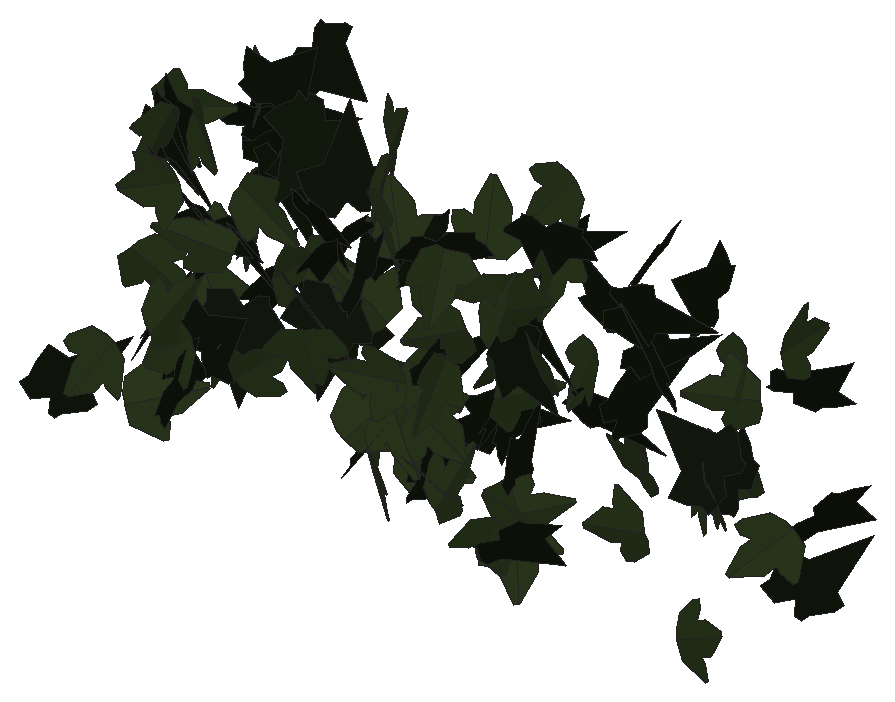
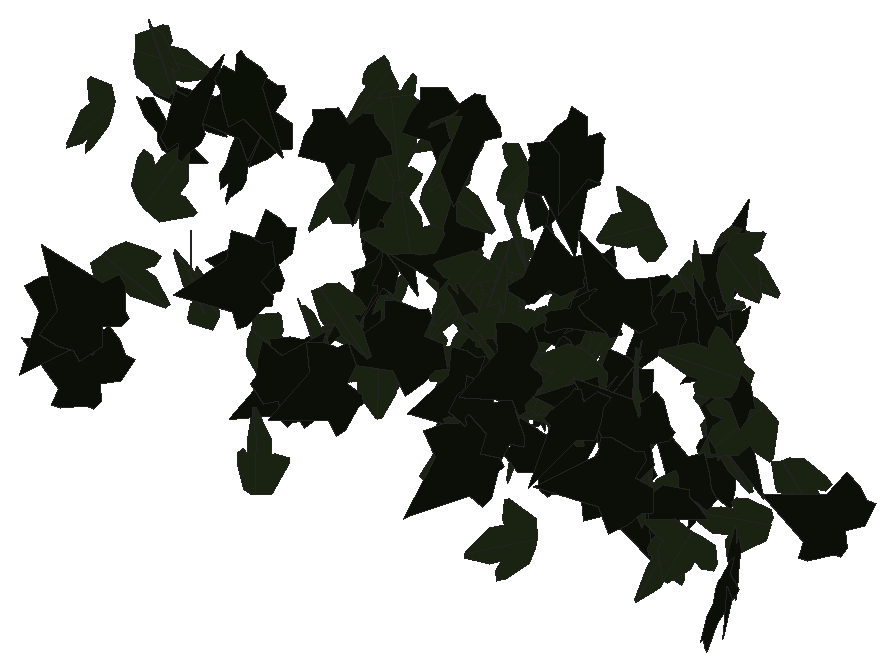
# SketchUp Ruby script. Lengths in inches.
U = 1.inch
M = Sketchup.active_model
def pt(a) = Geom::Point3d.new(a.map { |v| v * U })
def face(e, loops, mat)
  f = e.add_face(loops[0].map { |a| pt(a) })
  loops[1..].each { |l| e.add_face(l.map { |a| pt(a) }).erase! }
  f.material = f.back_material = mat if mat
  f
end
# faces: each face lists its corners as indices into pts; further lists are holes
def faces(e, pts, list, mat = nil) = list.each { |f| face(e, (f[0].is_a?(Array) ? f : [f]).map { |l| l.map { |i| pts[i] } }, mat) }
# xy, xz, yz: faces in a plane at the given z, y or x. An outline is a flat list of corners, or four numbers for a rectangle; further outlines are holes
def ring(l) = l.size == 4 ? [[l[0], l[1]], [l[2], l[1]], [l[2], l[3]], [l[0], l[3]]] : l.each_slice(2).to_a
def flat(e, list, mat, &to3) = list.each { |f| face(e, (f[0].is_a?(Array) ? f : [f]).map { |l| ring(l).map { |u, v| to3.(u, v) } }, mat) }
def xy(e, z, list, mat = nil) = flat(e, list, mat) { |x, y| [x, y, z] }
def xz(e, y, list, mat = nil) = flat(e, list, mat) { |x, z| [x, y, z] }
def yz(e, x, list, mat = nil) = flat(e, list, mat) { |y, z| [x, y, z] }
def lines(e, pts, list) = list.each { |a, b| e.add_line(pt(pts[a]), pt(pts[b])) }
# prism: a flat outline (further loops are holes) pulled along v
def prism(e, loops, v, mat = nil)
  f = face(e, loops, mat); d = Geom::Vector3d.new(v.map { |x| x * U })
  f.pushpull(f.normal.samedirection?(d) ? d.length : -d.length)
end
def box(e, o, s, mat = nil) = prism(e, [[o, [o[0] + s[0], o[1], o[2]], [o[0] + s[0], o[1] + s[1], o[2]], [o[0], o[1] + s[1], o[2]]]], [0, 0, s[2]], mat)
def at(x, y, z, deg = 0) = Geom::Transformation.translation(pt([x, y, z])) * Geom::Transformation.rotation(ORIGIN, Z_AXIS, deg.degrees)
def axes(o, x, y, z) = Geom::Transformation.new([*x, 0, *y, 0, *z, 0, *pt(o).to_a, 1])
def part(name) = M.definitions.add(name)
# library, detail: a bought-in or finely detailed component or shape, given as its bounding box
def library(name, o, s) = part(name).tap { |d| box(d.entities, o, s) }
def detail(e, o, s) = box(e.add_group.entities, o, s)
def put(e, d, t, mat = nil) = e.add_instance(d, t).tap { |i| i.material = mat if mat }
def group(e, t, mat = nil) = e.add_group.tap { |g| g.transformation = t; g.material = mat if mat }.entities
root = M.entities
M.materials.add("efeu1").color = [18, 25, 13]
M.materials.add("efeu2").color = [43, 57, 29]
c1 = part("ivyleaf_9")
p = [[1.54,2.16,1.25],[1.36,2.04,1.19],[-0.21,0.99,0.68],[-0.71,1.11,0.82],[-0.85,0.86,0.67],[-0.8,0.17,0.21],
  [-0.9,-0.01,0.1],[-0.67,-0.16,-0.02],[-0.08,-0.08,-0.05],[-0.03,-0.6,-0.4],[0.65,-0.88,-0.66],[0.83,-0.6,-0.49],
  [1.29,-0.42,-0.43],[1.8125,-0.07,-0.26],[1.21,0.44,0.15]]
faces(c1.entities,p,[[0,1,2,3,4,5,6,7,8,9,10,11,12,13,14]],"efeu1")
c2 = part("ivyleaf_10")
p = [[0,0.5,-0.03],[-0.0625,2.02,-0.43],[-0.19,2.01,-0.46],[-0.54,1.05,-0.29],[-0.52,0.625,-0.18],[-0.83,0.76,-0.28],
  [-1.16,0.64,-0.33],[-1.15,0.33,-0.24],[-0.77,-0.39,0.02],[-0.3,-0.51,0.16],[0.04,-0.48,0.23],[-0.02,2.01,-0.4375],
  [-0.06,2.01,-0.43],[0.04,-0.49,0.23],[0.67,-0.49,0.14],[1.38,0.36,-0.2],[1.375,0.51,-0.24],[0.81,0.65,-0.19],
  [0.62,0.59,-0.15],[0.6,1.09,-0.28],[0.5,1.23,-0.31]]
faces(c2.entities,p,[[0,1,2,3,4,5,6,7,8,9,10],[11,12,0,13,14,15,16,17,18,19,20]],"efeu2")
put(root,c1,axes([43.35,221.53,207.23],[0.45432,0.02484,-0.2073],[-0.20694,-0.0122,-0.455],[-0.02766,0.49923,-0.00081]))
put(root,c2,axes([46.76,221.66,202.9],[-0.31271,-0.38378,-0.07017],[0.04449,0.05425,-0.49505],[0.3876,-0.31586,0.00022]))
put(root,c1,axes([47.18,221.57,206.24],[0.2418,-0.30239,-0.31637],[-0.16835,0.26937,-0.38613],[0.40397,0.29325,0.02846]))
put(root,c2,axes([44.68,221.74,204.64],[0.03954,-0.01046,-0.49832],[-0.49747,0.03022,-0.04011],[0.03095,0.49898,-0.00802]))
put(root,c2,axes([45.54,221.95,204.97],[0.04865,0.35182,-0.35193],[-0.06472,-0.34613,-0.35497],[-0.4934,0.08009,0.01186]))
put(root,c2,axes([47.03,221.4,206.375],[0.00393,0.31947,-0.3846],[0.00224,0.3846,0.31949],[0.49998,-0.00424,0.00159]))
put(root,c2,axes([50.32,221.9,202.12],[0.19082,-0.11068,-0.44871],[0.37864,-0.2409,0.22044],[-0.26499,-0.42393,-0.00812]))
put(root,c2,axes([46.91,221.98,203.04],[-0.10747,0.34806,0.34249],[0.09946,-0.32774,0.36428],[0.47808,0.14643,0.00121]))
put(root,c2,axes([43.1,221.73,204.78],[-0.4383,-0.2361,-0.04633],[0.04211,0.01951,-0.49784],[0.23689,-0.44031,0.00278]))
put(root,c1,axes([43.75,221.61,206.77],[-0.04412,0.49157,-0.08007],[0.00277,-0.08014,-0.49353],[-0.49804,-0.04399,0.00434]))
put(root,c1,axes([51.04,221.76,205.26],[-0.41065,-0.14113,-0.24789],[-0.22963,-0.09422,0.43404],[-0.16923,0.47032,0.01257]))
put(root,c2,axes([39.1,221.83,203.12],[0.43051,-0.06518,-0.24579],[-0.2439,0.03088,-0.43539],[0.07194,0.49477,-0.00521]))
put(root,c1,axes([47.08,221.5,202.84],[0.33902,0.34548,0.12535],[0.08795,0.08933,-0.48403],[-0.35684,0.35024,-0.0002]))
put(root,c2,axes([40.33,221.78,206.49],[0.2199,-0.04325,-0.44696],[-0.42776,0.13124,-0.22315],[0.13662,0.48053,0.02072]))
put(root,c2,axes([46.66,222.07,205.55],[-0.10134,-0.41992,-0.25178],[0.01766,-0.26009,0.42666],[-0.4893,0.07759,0.06754]))
put(root,c1,axes([38.39,221.56,202.29],[-0.00687,-0.00369,0.49994],[0.45435,0.20859,0.00779],[-0.20862,0.4544,0.00049]))
put(root,c2,axes([45.56,221.92,206.91],[0.23152,0.42123,-0.1377],[-0.07114,-0.11802,-0.48064],[-0.43742,0.24215,0.00529]))
put(root,c2,axes([47.23,221.54,206.88],[-0.03633,-0.19491,-0.45901],[0.08664,0.45076,-0.19826],[0.49109,-0.09395,0.00102]))
put(root,c2,axes([47.11,221.5625,205.34],[-0.05853,-0.08283,-0.48961],[0.25997,0.41492,-0.10127],[0.42307,-0.26642,-0.0055]))
put(root,c2,axes([44.1,221.71,203.66],[0.2989,0.1501,-0.37166],[0.33203,0.167,0.33447],[0.22454,-0.44675,0.00016]))
put(root,c2,axes([45.74,222.01,205.75],[-0.18904,-0.08032,0.45587],[-0.4238,-0.16801,-0.20534],[0.18616,-0.46403,-0.00456]))
put(root,c2,axes([44.62,221.91,203.94],[0.41171,0.09001,0.26905],[0.25718,0.08181,-0.42091],[-0.11979,0.48498,0.02107]))
put(root,c2,axes([50.84,221.77,204.9375],[-0.35148,0.26985,0.23161],[-0.18644,0.13748,-0.4431],[-0.30283,-0.39784,0.00398]))
put(root,c1,axes([44.375,221.77,203.52],[-0.18094,0.46067,0.07101],[-0.03614,0.06208,-0.49481],[-0.46471,-0.1842,0.01083]))
put(root,c1,axes([46.89,221.98,205.07],[-0.2203,0.42523,-0.1437],[0.06215,-0.12963,-0.47889],[-0.44453,-0.22886,0.00426]))
put(root,c1,axes([44.19,221.77,206.21],[-0.29069,0.1354,-0.38363],[-0.34489,0.16804,0.32064],[0.21576,0.45103,-0.0043]))
put(root,c2,axes([45.32,221.82,204.18],[0.13161,0.36904,0.31062],[0.08006,0.3008,-0.39129],[-0.47568,0.15273,0.02008]))
put(root,c2,axes([46.59,222.11,206.79],[-0.31601,-0.38523,0.04169],[-0.02644,-0.03223,-0.49826],[0.38657,-0.31711,0]))
put(root,c2,axes([47.34,221.95,205.92],[-0.41901,0.18221,0.20305],[-0.18826,0.07623,-0.45689],[-0.19745,-0.45934,0.00473]))
put(root,c1,axes([45.48,221.93,207.2],[0.23324,0.40175,-0.18493],[-0.10128,-0.15499,-0.46446],[-0.43051,0.25412,0.00907]))
put(root,c1,axes([40.24,222.29,206.05],[0.3681,-0.32071,0.10794],[-0.07679,0.07616,0.48816],[-0.32956,-0.37596,0.00681]))
put(root,c2,axes([40.96,222.26,205.4],[0.12781,0.09886,0.47317],[-0.36591,-0.30004,0.16152],[0.31588,-0.38756,-0.00435]))
put(root,c2,axes([45.38,221.74,206.62],[-0.00296,0.20045,0.45805],[-0.08688,0.45089,-0.19787],[-0.49239,-0.08076,0.03216]))
put(root,c2,axes([41.72,222.11,206.57],[0.23522,0.03018,0.44018],[0.42187,0.13072,-0.23439],[-0.12923,0.48166,0.03603]))
put(root,c2,axes([40.2,221.82,204.07],[0.05586,0.16556,-0.46848],[0.13592,0.44835,0.17465],[0.47792,-0.14687,0.00508]))
put(root,c2,axes([51.05,222.35,206.31],[-0.03612,0.02668,0.49798],[-0.42886,-0.25647,-0.01737],[0.25451,-0.42838,0.04141]))
put(root,c1,axes([42.47,222.17,205.31],[0.45795,-0.19849,-0.02968],[-0.02765,0.01082,-0.49912],[0.19878,0.45879,-0.00106]))
put(root,c2,axes([46.86,221.93,203.03],[-0.00418,-0.00227,-0.49998],[0.36037,0.34657,-0.00458],[0.34658,-0.36039,-0.00126]))
put(root,c2,axes([46.74,222.22,202.44],[0.37811,0.32562,0.03165],[0.02367,0.02102,-0.499],[-0.3263,0.37885,0.00048]))
put(root,c1,axes([44.89,222,203.18],[0.45553,0.07713,-0.19117],[-0.2049,0.11841,-0.44045],[-0.02266,0.47961,0.13949]))
put(root,c2,axes([40.26,222.2,203.57],[0.35093,-0.12137,-0.33484],[-0.30124,0.14962,-0.36995],[0.19,0.46139,0.03189]))
put(root,c1,axes([51.08,222.1,204.9],[-0.1559,0.16793,0.4444],[-0.30212,0.32592,-0.22914],[-0.36664,-0.33997,-0.00015]))
put(root,c1,axes([40.39,221.97,203.05],[-0.05734,0.04993,-0.49419],[-0.34391,0.35494,0.07576],[0.35838,0.3486,-0.00636]))
put(root,c2,axes([45.51,221.96,202.85],[0.0448,0.20704,-0.45291],[0.06869,0.44782,0.21151],[0.49323,-0.08117,0.01168]))
put(root,c1,axes([40.89,222.28,205.79],[0.25536,0.2511,-0.34892],[-0.24352,-0.24994,-0.35809],[-0.35425,0.35282,-0.00535]))
put(root,c1,axes([45.28,221.99,204.74],[0.09046,0.08246,0.48479],[0.33107,0.35426,-0.12203],[-0.3636,0.34308,0.0095]))
put(root,c2,axes([44.73,222.29,204.32],[-0.42024,0.02271,0.26997],[-0.26948,0.01618,-0.42085],[-0.02785,-0.49922,-0.00136]))
put(root,c1,axes([39.98,222.38,204.125],[-0.25861,0.39169,-0.17233],[0.09915,-0.14103,-0.46934],[-0.41628,-0.27692,-0.00473]))
put(root,c2,axes([39.62,222.65,206.95],[0.0227,-0.41266,0.28142],[0.0645,-0.27693,-0.41128],[0.4953,0.05498,0.04066]))
put(root,c1,axes([46.85,222.09,203.54],[-0.001,-0.10231,0.48942],[0.14173,0.46929,0.09839],[-0.47949,0.13893,0.02807]))
put(root,c2,axes([44.93,222.18,204.7],[0.127,0.3496,0.33414],[0.0784,0.32602,-0.3709],[-0.47721,0.1466,0.02799]))
put(root,c2,axes([39.54,222.25,202.28],[0.15217,-0.04726,-0.47393],[0.43568,0.21481,0.11847],[0.19241,-0.44902,0.10656]))
put(root,c1,axes([42.85,222.75,204.83],[-0.13829,-0.48048,0.00368],[0.00553,-0.00542,-0.49994],[0.48046,-0.13824,0.00682]))
put(root,c2,axes([43.8,222.57,206.97],[-0.2793,0.28179,-0.30428],[0.2231,-0.20716,-0.39663],[-0.3496,-0.35733,-0.01002]))
put(root,c2,axes([50.74,222.54,206.79],[0.37861,-0.30443,-0.11824],[-0.09223,0.07398,-0.48582],[0.31329,0.38968,-0.00014]))
put(root,c1,axes([46.61,222.27,204.6],[0.01057,-0.02682,-0.49917],[-0.36277,0.3431,-0.02612],[0.34393,0.36272,-0.01221]))
put(root,c2,axes([43.75,222.54,202.62],[-0.33435,0.3712,-0.02055],[0.0117,-0.01712,-0.49957],[-0.37158,-0.33454,0.00276]))
put(root,c1,axes([40.91,222.59,205.55],[0.4846,-0.06703,-0.10328],[-0.1024,0.01348,-0.48922],[0.06837,0.4953,-0.00066]))
put(root,c1,axes([44.77,222.38,202.7],[0.11371,0.17084,0.45594],[0.24236,0.38623,-0.20516],[-0.4223,0.26766,0.00503]))
put(root,c2,axes([39.21,222.72,204.44],[-0.34769,-0.12366,-0.33737],[0.32457,0.09332,-0.36871],[0.15416,-0.47539,0.01538]))
put(root,c2,axes([50.53,222.91,204.39],[-0.43819,0.01177,-0.24052],[-0.24069,-0.00586,0.43821],[0.0075,0.49983,0.0108]))
put(root,c1,axes([42.6,223.08,203.96],[0.32253,-0.31868,0.21075],[0.15127,-0.14676,-0.45341],[0.35085,0.35624,0.00174]))
put(root,c1,axes([40.03,223.1,202.95],[-0.0824,0.07023,0.48814],[0.3284,-0.36141,0.10743],[0.36792,0.33831,0.01343]))
put(root,c2,axes([41.91,222.68,205.06],[-0.03297,0.07449,0.49332],[-0.22199,0.44057,-0.08136],[-0.4468,-0.22439,0.00403]))
put(root,c2,axes([39.77,223.23,206.67],[0.10338,-0.05558,0.48603],[0.45681,-0.16677,-0.11623],[0.17503,0.46808,0.0163]))
put(root,c2,axes([48.29,223.12,202.73],[-0.11113,-0.0061,0.48746],[-0.47878,-0.09276,-0.11031],[0.09178,-0.49128,0.01478]))
put(root,c1,axes([48.25,222.95,206.62],[0.14349,0.1607,-0.45121],[0.28659,0.34859,0.21529],[0.38377,-0.3204,0.00793]))
put(root,c1,axes([48.77,223.26,205.43],[0.16228,-0.413,0.23042],[-0.08615,0.21372,0.44374],[-0.46502,-0.18372,-0.00179]))
put(root,c1,axes([45.38,222.97,203.76],[0.0561,0.19887,-0.45531],[0.11246,0.44123,0.20657],[0.48395,-0.12559,0.00478]))
put(root,c2,axes([50.82,223.44,203.33],[0.34991,0.08396,-0.34715],[-0.33552,-0.0893,-0.35979],[-0.12242,0.48474,-0.00615]))
put(root,c2,axes([49.18,223.64,203.75],[0.18701,-0.12255,0.44722],[0.37118,-0.24948,-0.22357],[0.27795,0.41562,-0.00234]))
put(root,c2,axes([40.62,223.375,202.59],[-0.29338,-0.24097,0.32536],[0.3074,0.12892,0.37267],[-0.26349,0.41871,0.0725]))
put(root,c1,axes([46.43,223.35,207.15],[0.29596,0.27795,-0.29181],[-0.21379,-0.19861,-0.40601],[-0.34161,0.3651,0.00128]))
put(root,c1,axes([39.14,223.19,202.35],[0.05598,0.00361,-0.49684],[-0.44583,0.22106,-0.04862],[0.21932,0.44846,0.02797]))
put(root,c2,axes([43.05,223.65,206.83],[0.3196,-0.33938,0.18077],[0.12274,-0.13273,-0.46617],[0.36441,0.34235,-0.00154]))
put(root,c1,axes([48.42,223.54,207.43],[-0.27699,0.34379,-0.2347],[0.13049,-0.19598,-0.44109],[-0.39528,-0.30561,0.01885]))
put(root,c1,axes([38.92,223.52,206.14],[0.38501,-0.31829,0.0214],[0.01711,-0.01289,-0.49954],[0.31855,0.38539,0.00097]))
put(root,c2,axes([44.02,223.21,202.5],[0.10949,0.20576,0.44235],[0.21777,0.38507,-0.23302],[-0.43656,0.24369,-0.00529]))
put(root,c1,axes([38.93,223.9,206.01],[-0.05435,-0.00151,0.49703],[0.23458,-0.44089,0.02431],[0.4382,0.23583,0.04864]))
put(root,c2,axes([46.22,223.9,206.4],[0.06272,0.4199,-0.2641],[-0.04944,-0.25958,-0.42447],[-0.49358,0.07936,0.00896]))
put(root,c2,axes([42.82,223.79,204.3125],[0.28556,0.11974,0.39258],[-0.36074,-0.15488,0.30964],[0.19576,-0.46008,-0.00206]))
put(root,c1,axes([40.13,223.92,203.3],[-0.29861,-0.31825,-0.24403],[0.16508,0.17973,-0.4364],[0.36549,-0.34119,-0.00226]))
put(root,c1,axes([47.79,223.43,204.37],[0.04617,0.0739,0.49235],[0.3157,0.37799,-0.08634],[-0.38497,0.31884,-0.01176]))
put(root,c1,axes([42.25,223.77,206.07],[-0.30008,-0.2617,0.30243],[0.25311,0.16848,0.39693],[-0.30966,0.39132,0.03136]))
put(root,c1,axes([48.98,224.22,206.48],[0.02734,0.04289,0.49741],[-0.22872,-0.44172,0.05066],[0.44378,-0.2303,-0.00453]))
put(root,c1,axes([38.43,224,206.02],[-0.00634,-0.03686,-0.4986],[0.49062,0.09547,-0.0133],[0.09618,-0.48941,0.03496]))
put(root,c1,axes([38.55,224.4,202.2],[0.06636,-0.07855,-0.48931],[0.38793,-0.29898,0.1006],[-0.30839,-0.39299,0.02126]))
put(root,c1,axes([45.49,224.03,205.05],[0.40659,-0.24961,-0.14958],[-0.11926,0.09149,-0.47687],[0.26544,0.42347,0.01486]))
put(root,c1,axes([43.64,224.12,205.52],[-0.40173,0.29718,-0.01724],[0.01023,-0.01515,-0.49967],[-0.2975,-0.40181,0.0061]))
put(root,c2,axes([41.82,224.2,204.2],[0.46765,-0.17382,-0.03301],[-0.03107,0.01114,-0.49891],[0.17417,0.46868,-0.00038]))
put(root,c2,axes([44.74,224.04,206.08],[0.42707,0.254,-0.05565],[0.04074,0.04032,0.4967],[0.25681,-0.42879,0.01374]))
put(root,c2,axes([39.77,223.98,202.58],[-0.01733,-0.29155,-0.40583],[0.08761,0.39801,-0.28968],[0.49196,-0.08115,0.03729]))
put(root,c2,axes([41.41,224.14,204.51],[0.16688,0.02369,0.47073],[0.4171,0.22513,-0.15919],[-0.2195,0.44582,0.05537]))
put(root,c2,axes([42.88,224.22,205.35],[0.32736,0.37707,0.0256],[-0.01677,-0.01935,0.49934],[0.37756,-0.32779,-0.00002]))
put(root,c1,axes([41.98,224.33,203.25],[0.1108,-0.0026,0.48756],[-0.46597,0.14662,0.10667],[-0.14353,-0.47801,0.03007]))
put(root,c1,axes([41.07,224.67,206.51],[-0.2878,-0.40047,0.08242],[-0.04701,-0.06772,-0.49316],[0.40615,-0.29161,0.00133]))
put(root,c2,axes([38.54,224.22,206.1],[-0.09657,-0.0472,0.48831],[0.40876,0.26746,0.10669],[-0.27128,0.41981,-0.01307]))
put(root,c2,axes([50.64,224.03,206.27],[-0.00225,0.02415,0.49941],[-0.17396,0.46818,-0.02342],[-0.46876,-0.17386,0.00629]))
put(root,c2,axes([46.34,224.4375,204.375],[0.38491,-0.29434,-0.12333],[-0.09856,0.07413,-0.48455],[0.30353,0.39733,-0.00096]))
put(root,c2,axes([39.99,224.45,204.58],[0.184,-0.46066,-0.06272],[-0.02507,0.05752,-0.49605],[0.46424,0.18569,-0.00193]))
put(root,c1,axes([40.44,224.46,203.8125],[-0.08753,0.40582,-0.27865],[0.05492,-0.2732,-0.41514],[-0.48921,-0.10328,0.00325]))
put(root,c2,axes([39.0625,224.42,203.12],[0.4126,0.14846,0.24025],[0.2259,0.08179,-0.4385],[-0.1695,0.47039,0.00042]))
put(root,c1,axes([42.42,224.09,204.8],[0.12487,0.23638,0.42253],[0.219,0.36158,-0.26701],[-0.43179,0.25176,-0.01323]))
put(root,c1,axes([40.18,224.61,206.64],[-0.19585,0.00001,0.46005],[0.39411,-0.25792,0.16779],[0.23731,0.42834,0.10102]))
put(root,c1,axes([50.47,224.35,201.82],[-0.04466,-0.03213,0.49696],[0.46673,0.17133,0.05302],[-0.1737,0.46863,0.01469]))
put(root,c1,axes([40.14,224.8125,205.5],[0.24181,-0.42976,-0.0827],[-0.04043,0.07214,-0.49311],[0.43577,0.24516,0.00014]))
put(root,c1,axes([46.18,224.58,203.51],[0.47598,0.02525,0.151],[0.15109,0.00217,-0.47662],[-0.02472,0.49936,-0.00557]))
put(root,c1,axes([47.37,224.38,204.64],[0.16102,0.16478,0.44376],[0.32979,0.2972,-0.23002],[-0.33958,0.36677,-0.01297]))
put(root,c2,axes([42.17,224.5625,202.06],[0.05243,-0.09673,0.48774],[0.02826,0.49024,0.09418],[-0.49644,0.01769,0.05688]))
put(root,c1,axes([50.65,224.6,203.17],[0.23236,0.38628,0.21633],[0.11058,0.18593,-0.45078],[-0.4287,0.25733,0.00097]))
put(root,c2,axes([42.41,224.625,206.75],[0.06277,-0.04114,-0.49434],[-0.10373,0.48617,-0.05363],[0.48508,0.10929,0.0525]))
put(root,c1,axes([39.85,224.83,205.35],[0.23129,0.0557,0.43977],[0.42376,0.11783,-0.23779],[-0.13013,0.48271,0.0073]))
put(root,c1,axes([40.23,225.59,205.18],[0.20404,-0.35154,-0.29119],[0.15783,-0.24495,0.40631],[-0.42832,-0.25772,0.01101]))
put(root,c1,axes([42.41,224.91,204.45],[0.02239,0.48629,0.11409],[0.00387,0.11404,-0.48681],[-0.49948,0.02268,0.00134]))
put(root,c2,axes([39.17,225.51,206.17],[-0.04717,0.05067,0.49518],[0.38851,-0.3072,0.06845],[0.31118,0.39123,-0.01039]))
put(root,c2,axes([40.56,225.14,205.85],[-0.39331,-0.10354,-0.29083],[0.28037,0.07735,-0.4067],[0.12921,-0.48301,-0.00279]))
put(root,c2,axes([46.49,225.47,202.07],[-0.45645,0.07582,0.18949],[0.17987,-0.06996,0.46125],[0.09646,0.48924,0.03659]))
put(root,c2,axes([39.41,225.04,204.27],[0.07345,-0.11315,-0.48146],[-0.03021,0.4848,-0.11854],[0.49365,0.0465,0.06438]))
put(root,c1,axes([38.94,225.57,205.34],[0.36515,0.29813,-0.16668],[0.13034,0.10391,0.4714],[0.31572,-0.38771,-0.00183]))
put(root,c1,axes([42.08,225.72,204.08],[0.46663,0.15749,0.08636],[0.08057,0.03132,-0.49247],[-0.16053,0.47351,0.00385]))
put(root,c2,axes([44.6,226.05,206.02],[0.37993,-0.10639,-0.30714],[-0.29444,0.08749,-0.39453],[0.13769,0.48065,0.00383]))
put(root,c1,axes([49.06,226.08,204.08],[0.42494,0.24644,-0.09323],[0.07922,0.04923,0.49122],[0.25129,-0.43226,0.0028]))
put(root,c1,axes([45.52,226.15,204.06],[0.24191,-0.18842,0.39494],[-0.30741,0.24799,0.3066],[-0.31142,-0.39116,0.00414]))
put(root,c1,axes([38.72,226.22,205.09],[0.13247,0.21065,-0.43368],[0.12296,0.42012,0.24162],[0.46619,-0.17067,0.0595]))
put(root,c1,axes([44.3,226.14,204.71],[0.1887,0.25255,0.38809],[0.23532,0.30862,-0.31525],[-0.39877,0.30162,-0.00239]))
put(root,c1,axes([39.33,226.66,206.31],[0.10303,-0.19491,-0.44877],[-0.18454,0.40926,-0.22011],[0.45313,0.21099,0.0124]))
